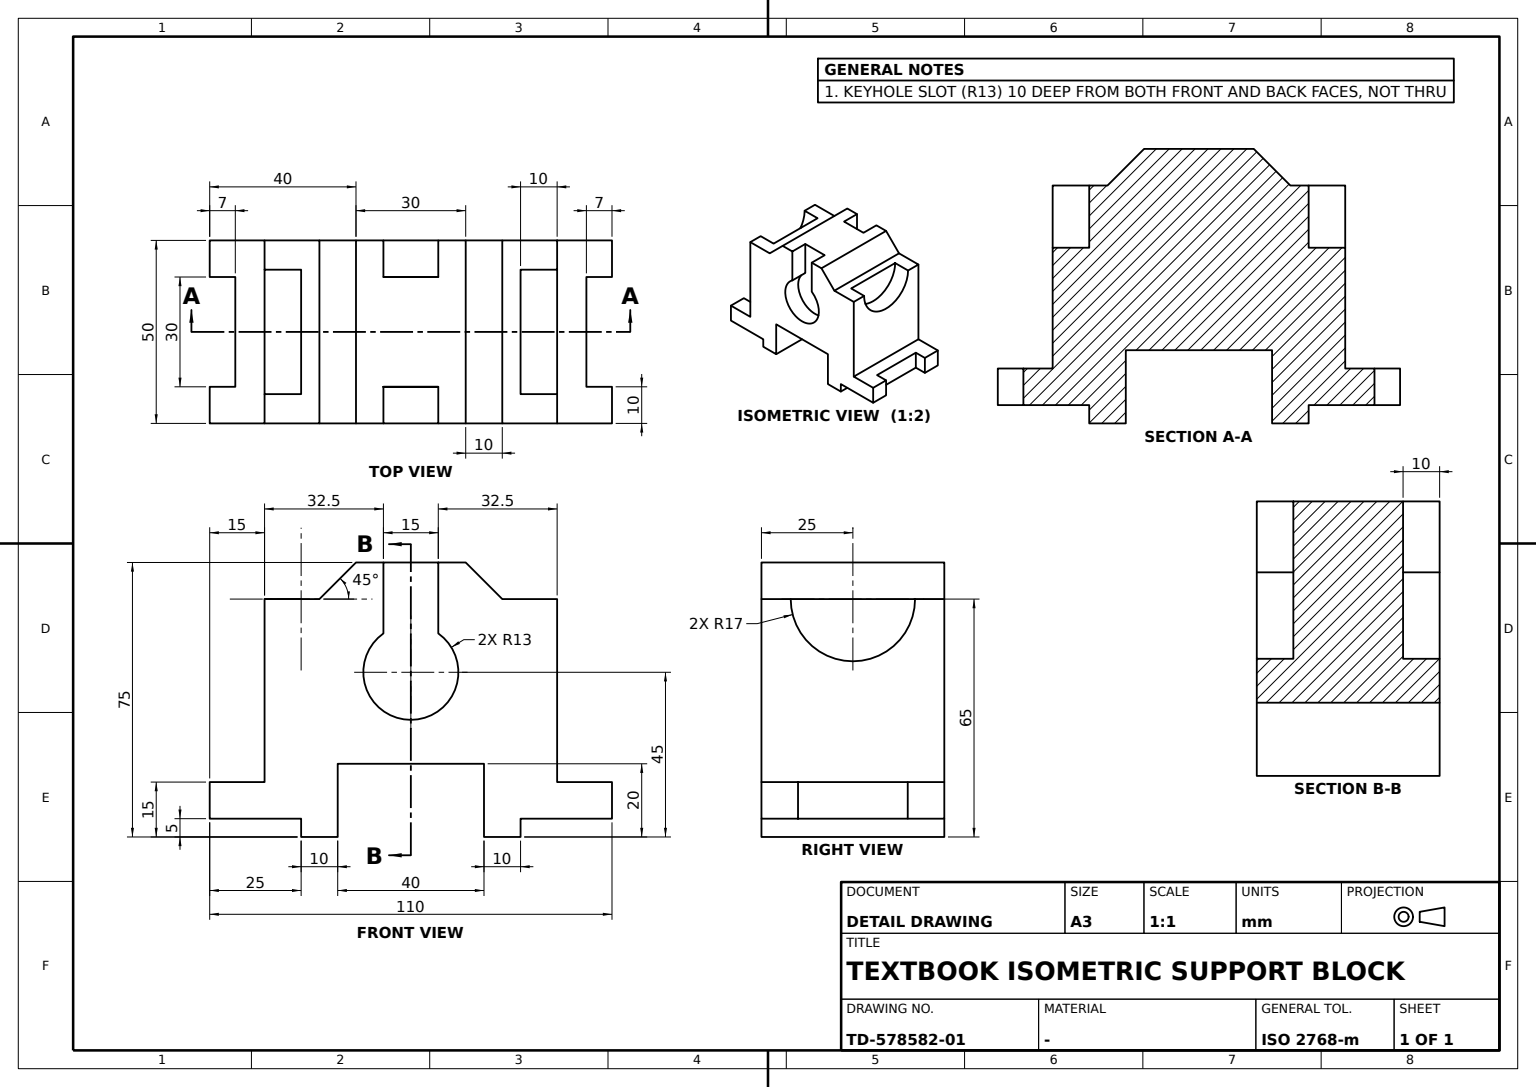
ISO-10303-21;
HEADER;
FILE_DESCRIPTION((''),'2;1');
FILE_NAME('','',(''),(''),'','','');
FILE_SCHEMA(('AUTOMOTIVE_DESIGN'));
ENDSEC;
DATA;
#1=APPLICATION_CONTEXT('');
#2=PRODUCT_CONTEXT('',#1,'mechanical');
#3=PRODUCT('','','',(#2));
#4=PRODUCT_DEFINITION_FORMATION('','',#3);
#5=PRODUCT_DEFINITION_CONTEXT('',#1,'design');
#6=PRODUCT_DEFINITION('','',#4,#5);
#7=PRODUCT_DEFINITION_SHAPE('','',#6);
#8=(LENGTH_UNIT()NAMED_UNIT(*)SI_UNIT(.MILLI.,.METRE.));
#9=(NAMED_UNIT(*)PLANE_ANGLE_UNIT()SI_UNIT($,.RADIAN.));
#10=(NAMED_UNIT(*)SI_UNIT($,.STERADIAN.)SOLID_ANGLE_UNIT());
#11=UNCERTAINTY_MEASURE_WITH_UNIT(LENGTH_MEASURE(0.005),#8,'distance_accuracy_value','');
#12=(GEOMETRIC_REPRESENTATION_CONTEXT(3)GLOBAL_UNCERTAINTY_ASSIGNED_CONTEXT((#11))GLOBAL_UNIT_ASSIGNED_CONTEXT((#8,#9,#10))REPRESENTATION_CONTEXT('',''));
#13=CARTESIAN_POINT('',(-78.,15.,5.));
#14=VERTEX_POINT('',#13);
#15=CARTESIAN_POINT('',(-78.,-15.,5.));
#16=VERTEX_POINT('',#15);
#17=CARTESIAN_POINT('',(-78.,0.,5.));
#18=DIRECTION('',(0.,-1.,0.));
#19=VECTOR('',#18,1000.);
#20=LINE('',#17,#19);
#21=EDGE_CURVE('',#14,#16,#20,.T.);
#22=ORIENTED_EDGE('',*,*,#21,.T.);
#23=CARTESIAN_POINT('',(-78.,-15.,15.));
#24=VERTEX_POINT('',#23);
#25=CARTESIAN_POINT('',(-78.,-15.,0.));
#26=DIRECTION('',(0.,0.,-1.));
#27=VECTOR('',#26,1000.);
#28=LINE('',#25,#27);
#29=EDGE_CURVE('',#24,#16,#28,.T.);
#30=ORIENTED_EDGE('',*,*,#29,.F.);
#31=CARTESIAN_POINT('',(-78.,15.,15.));
#32=VERTEX_POINT('',#31);
#33=LINE('',#31,#19);
#34=EDGE_CURVE('',#32,#24,#33,.T.);
#35=ORIENTED_EDGE('',*,*,#34,.F.);
#36=CARTESIAN_POINT('',(-78.,15.,0.));
#37=LINE('',#36,#27);
#38=EDGE_CURVE('',#32,#14,#37,.T.);
#39=ORIENTED_EDGE('',*,*,#38,.T.);
#40=EDGE_LOOP('',(#22,#30,#35,#39));
#41=FACE_BOUND('',#40,.T.);
#42=DIRECTION('',(1.,0.,0.));
#43=AXIS2_PLACEMENT_3D('',#31,#42,#18);
#44=PLANE('',#43);
#45=ADVANCED_FACE('',(#41),#44,.F.);
#46=ORIENTED_EDGE('',*,*,#21,.F.);
#47=CARTESIAN_POINT('',(-85.,15.,5.));
#48=VERTEX_POINT('',#47);
#49=CARTESIAN_POINT('',(0.,15.,5.));
#50=DIRECTION('',(-1.,0.,0.));
#51=VECTOR('',#50,1000.);
#52=LINE('',#49,#51);
#53=EDGE_CURVE('',#14,#48,#52,.T.);
#54=ORIENTED_EDGE('',*,*,#53,.T.);
#55=CARTESIAN_POINT('',(-85.,25.,5.));
#56=VERTEX_POINT('',#55);
#57=CARTESIAN_POINT('',(-85.,0.,5.));
#58=DIRECTION('',(0.,1.,0.));
#59=VECTOR('',#58,1000.);
#60=LINE('',#57,#59);
#61=EDGE_CURVE('',#48,#56,#60,.T.);
#62=ORIENTED_EDGE('',*,*,#61,.T.);
#63=CARTESIAN_POINT('',(-60.,25.,5.));
#64=VERTEX_POINT('',#63);
#65=CARTESIAN_POINT('',(0.,25.,5.));
#66=LINE('',#65,#51);
#67=EDGE_CURVE('',#64,#56,#66,.T.);
#68=ORIENTED_EDGE('',*,*,#67,.F.);
#69=CARTESIAN_POINT('',(-60.,-25.,5.));
#70=VERTEX_POINT('',#69);
#71=CARTESIAN_POINT('',(-60.,0.,5.));
#72=LINE('',#71,#59);
#73=EDGE_CURVE('',#70,#64,#72,.T.);
#74=ORIENTED_EDGE('',*,*,#73,.F.);
#75=CARTESIAN_POINT('',(-85.,-25.,5.));
#76=VERTEX_POINT('',#75);
#77=CARTESIAN_POINT('',(0.,-25.,5.));
#78=LINE('',#77,#51);
#79=EDGE_CURVE('',#70,#76,#78,.T.);
#80=ORIENTED_EDGE('',*,*,#79,.T.);
#81=CARTESIAN_POINT('',(-85.,-15.,5.));
#82=VERTEX_POINT('',#81);
#83=EDGE_CURVE('',#76,#82,#60,.T.);
#84=ORIENTED_EDGE('',*,*,#83,.T.);
#85=CARTESIAN_POINT('',(25.,-15.,5.));
#86=VECTOR('',#42,1000.);
#87=LINE('',#85,#86);
#88=EDGE_CURVE('',#82,#16,#87,.T.);
#89=ORIENTED_EDGE('',*,*,#88,.T.);
#90=EDGE_LOOP('',(#46,#54,#62,#68,#74,#80,#84,#89));
#91=FACE_BOUND('',#90,.T.);
#92=CARTESIAN_POINT('',(25.,0.,5.));
#93=AXIS2_PLACEMENT_3D('',#92,#26,#50);
#94=PLANE('',#93);
#95=ADVANCED_FACE('',(#91),#94,.T.);
#96=CARTESIAN_POINT('',(10.,-17.,65.));
#97=VERTEX_POINT('',#96);
#98=CARTESIAN_POINT('',(10.,17.,65.));
#99=VERTEX_POINT('',#98);
#100=CARTESIAN_POINT('',(10.,0.,65.));
#101=DIRECTION('',(0.,0.,1.));
#102=AXIS2_PLACEMENT_3D('',#100,#50,#101);
#103=CIRCLE('',#102,17.);
#104=EDGE_CURVE('',#97,#99,#103,.F.);
#105=ORIENTED_EDGE('',*,*,#104,.F.);
#106=CARTESIAN_POINT('',(10.,-25.,65.));
#107=VERTEX_POINT('',#106);
#108=LINE('',#100,#59);
#109=EDGE_CURVE('',#107,#97,#108,.T.);
#110=ORIENTED_EDGE('',*,*,#109,.F.);
#111=CARTESIAN_POINT('',(10.,-25.,15.));
#112=VERTEX_POINT('',#111);
#113=CARTESIAN_POINT('',(10.,-25.,0.));
#114=VECTOR('',#101,1000.);
#115=LINE('',#113,#114);
#116=EDGE_CURVE('',#112,#107,#115,.T.);
#117=ORIENTED_EDGE('',*,*,#116,.F.);
#118=CARTESIAN_POINT('',(10.,25.,15.));
#119=VERTEX_POINT('',#118);
#120=CARTESIAN_POINT('',(10.,0.,15.));
#121=LINE('',#120,#59);
#122=EDGE_CURVE('',#112,#119,#121,.T.);
#123=ORIENTED_EDGE('',*,*,#122,.T.);
#124=CARTESIAN_POINT('',(10.,25.,65.));
#125=VERTEX_POINT('',#124);
#126=CARTESIAN_POINT('',(10.,25.,0.));
#127=LINE('',#126,#114);
#128=EDGE_CURVE('',#119,#125,#127,.T.);
#129=ORIENTED_EDGE('',*,*,#128,.T.);
#130=EDGE_CURVE('',#99,#125,#108,.T.);
#131=ORIENTED_EDGE('',*,*,#130,.F.);
#132=EDGE_LOOP('',(#105,#110,#117,#123,#129,#131));
#133=FACE_BOUND('',#132,.T.);
#134=AXIS2_PLACEMENT_3D('',#120,#50,#101);
#135=PLANE('',#134);
#136=ADVANCED_FACE('',(#133),#135,.F.);
#137=CARTESIAN_POINT('',(-22.5,-15.,75.));
#138=VERTEX_POINT('',#137);
#139=CARTESIAN_POINT('',(-22.5,-15.,55.61838));
#140=VERTEX_POINT('',#139);
#141=LINE('',#137,#27);
#142=EDGE_CURVE('',#138,#140,#141,.T.);
#143=ORIENTED_EDGE('',*,*,#142,.T.);
#144=CARTESIAN_POINT('',(-22.5,-25.,55.61838));
#145=VERTEX_POINT('',#144);
#146=LINE('',#144,#59);
#147=EDGE_CURVE('',#145,#140,#146,.T.);
#148=ORIENTED_EDGE('',*,*,#147,.F.);
#149=CARTESIAN_POINT('',(-22.5,-25.,75.));
#150=VERTEX_POINT('',#149);
#151=LINE('',#149,#27);
#152=EDGE_CURVE('',#150,#145,#151,.T.);
#153=ORIENTED_EDGE('',*,*,#152,.F.);
#154=CARTESIAN_POINT('',(-22.5,0.,75.));
#155=LINE('',#154,#59);
#156=EDGE_CURVE('',#150,#138,#155,.T.);
#157=ORIENTED_EDGE('',*,*,#156,.T.);
#158=EDGE_LOOP('',(#143,#148,#153,#157));
#159=FACE_BOUND('',#158,.T.);
#160=CARTESIAN_POINT('',(-22.5,25.,75.));
#161=AXIS2_PLACEMENT_3D('',#160,#50,#26);
#162=PLANE('',#161);
#163=ADVANCED_FACE('',(#159),#162,.T.);
#164=CARTESIAN_POINT('',(-22.5,15.,55.61838));
#165=VERTEX_POINT('',#164);
#166=CARTESIAN_POINT('',(-37.5,15.,55.61838));
#167=VERTEX_POINT('',#166);
#168=CARTESIAN_POINT('',(-30.,15.,45.));
#169=AXIS2_PLACEMENT_3D('',#168,#58,#101);
#170=CIRCLE('',#169,13.);
#171=EDGE_CURVE('',#165,#167,#170,.T.);
#172=ORIENTED_EDGE('',*,*,#171,.F.);
#173=CARTESIAN_POINT('',(-22.5,25.,55.61838));
#174=VERTEX_POINT('',#173);
#175=LINE('',#173,#59);
#176=EDGE_CURVE('',#174,#165,#175,.F.);
#177=ORIENTED_EDGE('',*,*,#176,.F.);
#178=CARTESIAN_POINT('',(-37.5,25.,55.61838));
#179=VERTEX_POINT('',#178);
#180=CARTESIAN_POINT('',(-30.,25.,45.));
#181=AXIS2_PLACEMENT_3D('',#180,#58,#101);
#182=CIRCLE('',#181,13.);
#183=EDGE_CURVE('',#174,#179,#182,.T.);
#184=ORIENTED_EDGE('',*,*,#183,.T.);
#185=LINE('',#178,#59);
#186=EDGE_CURVE('',#179,#167,#185,.F.);
#187=ORIENTED_EDGE('',*,*,#186,.T.);
#188=EDGE_LOOP('',(#172,#177,#184,#187));
#189=FACE_BOUND('',#188,.T.);
#190=CARTESIAN_POINT('',(-30.,20.,45.));
#191=AXIS2_PLACEMENT_3D('',#190,#58,#50);
#192=CYLINDRICAL_SURFACE('',#191,13.);
#193=ADVANCED_FACE('',(#189),#192,.F.);
#194=CARTESIAN_POINT('',(-37.5,-15.,75.));
#195=VERTEX_POINT('',#194);
#196=CARTESIAN_POINT('',(0.,-15.,75.));
#197=LINE('',#196,#51);
#198=EDGE_CURVE('',#138,#195,#197,.T.);
#199=ORIENTED_EDGE('',*,*,#198,.T.);
#200=CARTESIAN_POINT('',(-37.5,-15.,55.61838));
#201=VERTEX_POINT('',#200);
#202=LINE('',#200,#114);
#203=EDGE_CURVE('',#201,#195,#202,.T.);
#204=ORIENTED_EDGE('',*,*,#203,.F.);
#205=CARTESIAN_POINT('',(-30.,-15.,45.));
#206=AXIS2_PLACEMENT_3D('',#205,#58,#101);
#207=CIRCLE('',#206,13.);
#208=EDGE_CURVE('',#140,#201,#207,.T.);
#209=ORIENTED_EDGE('',*,*,#208,.F.);
#210=ORIENTED_EDGE('',*,*,#142,.F.);
#211=EDGE_LOOP('',(#199,#204,#209,#210));
#212=FACE_BOUND('',#211,.T.);
#213=CARTESIAN_POINT('',(0.,-15.,0.));
#214=AXIS2_PLACEMENT_3D('',#213,#58,#50);
#215=PLANE('',#214);
#216=ADVANCED_FACE('',(#212),#215,.F.);
#217=CARTESIAN_POINT('',(25.,-25.,15.));
#218=VERTEX_POINT('',#217);
#219=CARTESIAN_POINT('',(25.,-15.,15.));
#220=VERTEX_POINT('',#219);
#221=CARTESIAN_POINT('',(25.,0.,15.));
#222=LINE('',#221,#59);
#223=EDGE_CURVE('',#218,#220,#222,.T.);
#224=ORIENTED_EDGE('',*,*,#223,.T.);
#225=CARTESIAN_POINT('',(18.,-15.,15.));
#226=VERTEX_POINT('',#225);
#227=CARTESIAN_POINT('',(-85.,-15.,15.));
#228=LINE('',#227,#51);
#229=EDGE_CURVE('',#220,#226,#228,.T.);
#230=ORIENTED_EDGE('',*,*,#229,.T.);
#231=CARTESIAN_POINT('',(18.,15.,15.));
#232=VERTEX_POINT('',#231);
#233=LINE('',#231,#19);
#234=EDGE_CURVE('',#232,#226,#233,.T.);
#235=ORIENTED_EDGE('',*,*,#234,.F.);
#236=CARTESIAN_POINT('',(25.,15.,15.));
#237=VERTEX_POINT('',#236);
#238=CARTESIAN_POINT('',(0.,15.,15.));
#239=LINE('',#238,#86);
#240=EDGE_CURVE('',#232,#237,#239,.T.);
#241=ORIENTED_EDGE('',*,*,#240,.T.);
#242=CARTESIAN_POINT('',(25.,25.,15.));
#243=VERTEX_POINT('',#242);
#244=EDGE_CURVE('',#237,#243,#222,.T.);
#245=ORIENTED_EDGE('',*,*,#244,.T.);
#246=CARTESIAN_POINT('',(-85.,25.,15.));
#247=LINE('',#246,#51);
#248=EDGE_CURVE('',#243,#119,#247,.T.);
#249=ORIENTED_EDGE('',*,*,#248,.T.);
#250=ORIENTED_EDGE('',*,*,#122,.F.);
#251=CARTESIAN_POINT('',(-85.,-25.,15.));
#252=LINE('',#251,#51);
#253=EDGE_CURVE('',#218,#112,#252,.T.);
#254=ORIENTED_EDGE('',*,*,#253,.F.);
#255=EDGE_LOOP('',(#224,#230,#235,#241,#245,#249,#250,#254));
#256=FACE_BOUND('',#255,.T.);
#257=CARTESIAN_POINT('',(-85.,0.,15.));
#258=AXIS2_PLACEMENT_3D('',#257,#101,#42);
#259=PLANE('',#258);
#260=ADVANCED_FACE('',(#256),#259,.T.);
#261=CARTESIAN_POINT('',(-60.,17.,65.));
#262=VERTEX_POINT('',#261);
#263=CARTESIAN_POINT('',(-60.,-17.,65.));
#264=VERTEX_POINT('',#263);
#265=CARTESIAN_POINT('',(-60.,0.,65.));
#266=AXIS2_PLACEMENT_3D('',#265,#50,#101);
#267=CIRCLE('',#266,17.);
#268=EDGE_CURVE('',#262,#264,#267,.T.);
#269=ORIENTED_EDGE('',*,*,#268,.T.);
#270=LINE('',#265,#19);
#271=EDGE_CURVE('',#262,#264,#270,.T.);
#272=ORIENTED_EDGE('',*,*,#271,.F.);
#273=EDGE_LOOP('',(#269,#272));
#274=FACE_BOUND('',#273,.T.);
#275=CARTESIAN_POINT('',(-60.,0.,0.));
#276=AXIS2_PLACEMENT_3D('',#275,#50,#101);
#277=PLANE('',#276);
#278=ADVANCED_FACE('',(#274),#277,.T.);
#279=CARTESIAN_POINT('',(-37.5,25.,75.));
#280=VERTEX_POINT('',#279);
#281=LINE('',#178,#114);
#282=EDGE_CURVE('',#179,#280,#281,.T.);
#283=ORIENTED_EDGE('',*,*,#282,.T.);
#284=CARTESIAN_POINT('',(-37.5,15.,75.));
#285=VERTEX_POINT('',#284);
#286=CARTESIAN_POINT('',(-37.5,0.,75.));
#287=LINE('',#286,#19);
#288=EDGE_CURVE('',#280,#285,#287,.T.);
#289=ORIENTED_EDGE('',*,*,#288,.T.);
#290=LINE('',#166,#114);
#291=EDGE_CURVE('',#167,#285,#290,.T.);
#292=ORIENTED_EDGE('',*,*,#291,.F.);
#293=ORIENTED_EDGE('',*,*,#186,.F.);
#294=EDGE_LOOP('',(#283,#289,#292,#293));
#295=FACE_BOUND('',#294,.T.);
#296=AXIS2_PLACEMENT_3D('',#178,#42,#101);
#297=PLANE('',#296);
#298=ADVANCED_FACE('',(#295),#297,.T.);
#299=CARTESIAN_POINT('',(18.,15.,5.));
#300=VERTEX_POINT('',#299);
#301=CARTESIAN_POINT('',(18.,-15.,5.));
#302=VERTEX_POINT('',#301);
#303=CARTESIAN_POINT('',(18.,0.,5.));
#304=LINE('',#303,#19);
#305=EDGE_CURVE('',#300,#302,#304,.T.);
#306=ORIENTED_EDGE('',*,*,#305,.F.);
#307=CARTESIAN_POINT('',(18.,15.,0.));
#308=LINE('',#307,#27);
#309=EDGE_CURVE('',#232,#300,#308,.T.);
#310=ORIENTED_EDGE('',*,*,#309,.F.);
#311=ORIENTED_EDGE('',*,*,#234,.T.);
#312=CARTESIAN_POINT('',(18.,-15.,0.));
#313=LINE('',#312,#27);
#314=EDGE_CURVE('',#226,#302,#313,.T.);
#315=ORIENTED_EDGE('',*,*,#314,.T.);
#316=EDGE_LOOP('',(#306,#310,#311,#315));
#317=FACE_BOUND('',#316,.T.);
#318=AXIS2_PLACEMENT_3D('',#231,#42,#18);
#319=PLANE('',#318);
#320=ADVANCED_FACE('',(#317),#319,.T.);
#321=VERTEX_POINT('',#160);
#322=LINE('',#160,#27);
#323=EDGE_CURVE('',#321,#174,#322,.T.);
#324=ORIENTED_EDGE('',*,*,#323,.T.);
#325=ORIENTED_EDGE('',*,*,#176,.T.);
#326=CARTESIAN_POINT('',(-22.5,15.,75.));
#327=VERTEX_POINT('',#326);
#328=LINE('',#326,#27);
#329=EDGE_CURVE('',#327,#165,#328,.T.);
#330=ORIENTED_EDGE('',*,*,#329,.F.);
#331=LINE('',#160,#19);
#332=EDGE_CURVE('',#321,#327,#331,.T.);
#333=ORIENTED_EDGE('',*,*,#332,.F.);
#334=EDGE_LOOP('',(#324,#325,#330,#333));
#335=FACE_BOUND('',#334,.T.);
#336=ADVANCED_FACE('',(#335),#162,.T.);
#337=CARTESIAN_POINT('',(25.,-25.,5.));
#338=VERTEX_POINT('',#337);
#339=VERTEX_POINT('',#77);
#340=EDGE_CURVE('',#338,#339,#78,.T.);
#341=ORIENTED_EDGE('',*,*,#340,.T.);
#342=VERTEX_POINT('',#65);
#343=CARTESIAN_POINT('',(0.,0.,5.));
#344=LINE('',#343,#59);
#345=EDGE_CURVE('',#339,#342,#344,.T.);
#346=ORIENTED_EDGE('',*,*,#345,.T.);
#347=CARTESIAN_POINT('',(25.,25.,5.));
#348=VERTEX_POINT('',#347);
#349=EDGE_CURVE('',#348,#342,#66,.T.);
#350=ORIENTED_EDGE('',*,*,#349,.F.);
#351=CARTESIAN_POINT('',(25.,15.,5.));
#352=VERTEX_POINT('',#351);
#353=LINE('',#92,#59);
#354=EDGE_CURVE('',#352,#348,#353,.T.);
#355=ORIENTED_EDGE('',*,*,#354,.F.);
#356=LINE('',#351,#86);
#357=EDGE_CURVE('',#300,#352,#356,.T.);
#358=ORIENTED_EDGE('',*,*,#357,.F.);
#359=ORIENTED_EDGE('',*,*,#305,.T.);
#360=VERTEX_POINT('',#85);
#361=CARTESIAN_POINT('',(0.,-15.,5.));
#362=LINE('',#361,#51);
#363=EDGE_CURVE('',#360,#302,#362,.T.);
#364=ORIENTED_EDGE('',*,*,#363,.F.);
#365=EDGE_CURVE('',#338,#360,#353,.T.);
#366=ORIENTED_EDGE('',*,*,#365,.F.);
#367=EDGE_LOOP('',(#341,#346,#350,#355,#358,#359,#364,#366));
#368=FACE_BOUND('',#367,.T.);
#369=ADVANCED_FACE('',(#368),#94,.T.);
#370=CARTESIAN_POINT('',(-70.,17.,65.));
#371=VERTEX_POINT('',#370);
#372=CARTESIAN_POINT('',(-70.,25.,65.));
#373=VERTEX_POINT('',#372);
#374=CARTESIAN_POINT('',(-70.,0.,65.));
#375=LINE('',#374,#59);
#376=EDGE_CURVE('',#371,#373,#375,.T.);
#377=ORIENTED_EDGE('',*,*,#376,.T.);
#378=CARTESIAN_POINT('',(-70.,25.,15.));
#379=VERTEX_POINT('',#378);
#380=CARTESIAN_POINT('',(-70.,25.,0.));
#381=LINE('',#380,#114);
#382=EDGE_CURVE('',#379,#373,#381,.T.);
#383=ORIENTED_EDGE('',*,*,#382,.F.);
#384=CARTESIAN_POINT('',(-70.,-25.,15.));
#385=VERTEX_POINT('',#384);
#386=CARTESIAN_POINT('',(-70.,0.,15.));
#387=LINE('',#386,#59);
#388=EDGE_CURVE('',#385,#379,#387,.T.);
#389=ORIENTED_EDGE('',*,*,#388,.F.);
#390=CARTESIAN_POINT('',(-70.,-25.,65.));
#391=VERTEX_POINT('',#390);
#392=CARTESIAN_POINT('',(-70.,-25.,0.));
#393=LINE('',#392,#114);
#394=EDGE_CURVE('',#385,#391,#393,.T.);
#395=ORIENTED_EDGE('',*,*,#394,.T.);
#396=CARTESIAN_POINT('',(-70.,-17.,65.));
#397=VERTEX_POINT('',#396);
#398=EDGE_CURVE('',#391,#397,#375,.T.);
#399=ORIENTED_EDGE('',*,*,#398,.T.);
#400=AXIS2_PLACEMENT_3D('',#374,#50,#101);
#401=CIRCLE('',#400,17.);
#402=EDGE_CURVE('',#371,#397,#401,.T.);
#403=ORIENTED_EDGE('',*,*,#402,.F.);
#404=EDGE_LOOP('',(#377,#383,#389,#395,#399,#403));
#405=FACE_BOUND('',#404,.T.);
#406=AXIS2_PLACEMENT_3D('',#386,#50,#101);
#407=PLANE('',#406);
#408=ADVANCED_FACE('',(#405),#407,.T.);
#409=ORIENTED_EDGE('',*,*,#329,.T.);
#410=ORIENTED_EDGE('',*,*,#171,.T.);
#411=ORIENTED_EDGE('',*,*,#291,.T.);
#412=CARTESIAN_POINT('',(0.,15.,75.));
#413=LINE('',#412,#51);
#414=EDGE_CURVE('',#327,#285,#413,.T.);
#415=ORIENTED_EDGE('',*,*,#414,.F.);
#416=EDGE_LOOP('',(#409,#410,#411,#415));
#417=FACE_BOUND('',#416,.T.);
#418=CARTESIAN_POINT('',(0.,15.,0.));
#419=AXIS2_PLACEMENT_3D('',#418,#58,#50);
#420=PLANE('',#419);
#421=ADVANCED_FACE('',(#417),#420,.T.);
#422=ORIENTED_EDGE('',*,*,#365,.T.);
#423=CARTESIAN_POINT('',(25.,-15.,0.));
#424=LINE('',#423,#27);
#425=EDGE_CURVE('',#220,#360,#424,.T.);
#426=ORIENTED_EDGE('',*,*,#425,.F.);
#427=ORIENTED_EDGE('',*,*,#223,.F.);
#428=CARTESIAN_POINT('',(25.,-25.,0.));
#429=LINE('',#428,#27);
#430=EDGE_CURVE('',#218,#338,#429,.T.);
#431=ORIENTED_EDGE('',*,*,#430,.T.);
#432=EDGE_LOOP('',(#422,#426,#427,#431));
#433=FACE_BOUND('',#432,.T.);
#434=AXIS2_PLACEMENT_3D('',#221,#42,#26);
#435=PLANE('',#434);
#436=ADVANCED_FACE('',(#433),#435,.T.);
#437=ORIENTED_EDGE('',*,*,#83,.F.);
#438=VERTEX_POINT('',#251);
#439=CARTESIAN_POINT('',(-85.,-25.,0.));
#440=LINE('',#439,#114);
#441=EDGE_CURVE('',#76,#438,#440,.T.);
#442=ORIENTED_EDGE('',*,*,#441,.T.);
#443=VERTEX_POINT('',#227);
#444=LINE('',#257,#59);
#445=EDGE_CURVE('',#438,#443,#444,.T.);
#446=ORIENTED_EDGE('',*,*,#445,.T.);
#447=LINE('',#81,#27);
#448=EDGE_CURVE('',#443,#82,#447,.T.);
#449=ORIENTED_EDGE('',*,*,#448,.T.);
#450=EDGE_LOOP('',(#437,#442,#446,#449));
#451=FACE_BOUND('',#450,.T.);
#452=AXIS2_PLACEMENT_3D('',#57,#50,#101);
#453=PLANE('',#452);
#454=ADVANCED_FACE('',(#451),#453,.T.);
#455=ORIENTED_EDGE('',*,*,#349,.T.);
#456=CARTESIAN_POINT('',(0.,25.,0.));
#457=VERTEX_POINT('',#456);
#458=LINE('',#456,#27);
#459=EDGE_CURVE('',#342,#457,#458,.T.);
#460=ORIENTED_EDGE('',*,*,#459,.T.);
#461=CARTESIAN_POINT('',(-10.,25.,0.));
#462=VERTEX_POINT('',#461);
#463=LINE('',#456,#51);
#464=EDGE_CURVE('',#457,#462,#463,.T.);
#465=ORIENTED_EDGE('',*,*,#464,.T.);
#466=CARTESIAN_POINT('',(-10.,25.,20.));
#467=VERTEX_POINT('',#466);
#468=LINE('',#461,#114);
#469=EDGE_CURVE('',#462,#467,#468,.T.);
#470=ORIENTED_EDGE('',*,*,#469,.T.);
#471=CARTESIAN_POINT('',(-50.,25.,20.));
#472=VERTEX_POINT('',#471);
#473=CARTESIAN_POINT('',(0.,25.,20.));
#474=LINE('',#473,#51);
#475=EDGE_CURVE('',#467,#472,#474,.T.);
#476=ORIENTED_EDGE('',*,*,#475,.T.);
#477=CARTESIAN_POINT('',(-50.,25.,0.));
#478=VERTEX_POINT('',#477);
#479=LINE('',#477,#27);
#480=EDGE_CURVE('',#472,#478,#479,.T.);
#481=ORIENTED_EDGE('',*,*,#480,.T.);
#482=CARTESIAN_POINT('',(-60.,25.,0.));
#483=VERTEX_POINT('',#482);
#484=EDGE_CURVE('',#478,#483,#463,.T.);
#485=ORIENTED_EDGE('',*,*,#484,.T.);
#486=LINE('',#482,#114);
#487=EDGE_CURVE('',#483,#64,#486,.T.);
#488=ORIENTED_EDGE('',*,*,#487,.T.);
#489=ORIENTED_EDGE('',*,*,#67,.T.);
#490=VERTEX_POINT('',#246);
#491=CARTESIAN_POINT('',(-85.,25.,0.));
#492=LINE('',#491,#114);
#493=EDGE_CURVE('',#56,#490,#492,.T.);
#494=ORIENTED_EDGE('',*,*,#493,.T.);
#495=CARTESIAN_POINT('',(0.,25.,15.));
#496=LINE('',#495,#86);
#497=EDGE_CURVE('',#490,#379,#496,.T.);
#498=ORIENTED_EDGE('',*,*,#497,.T.);
#499=ORIENTED_EDGE('',*,*,#382,.T.);
#500=CARTESIAN_POINT('',(-55.,25.,65.));
#501=VERTEX_POINT('',#500);
#502=CARTESIAN_POINT('',(0.,25.,65.));
#503=LINE('',#502,#86);
#504=EDGE_CURVE('',#373,#501,#503,.T.);
#505=ORIENTED_EDGE('',*,*,#504,.T.);
#506=CARTESIAN_POINT('',(-45.,25.,75.));
#507=VERTEX_POINT('',#506);
#508=CARTESIAN_POINT('',(-60.,25.,60.));
#509=DIRECTION('',(0.707106781,0.,0.707106781));
#510=VECTOR('',#509,1000.);
#511=LINE('',#508,#510);
#512=EDGE_CURVE('',#501,#507,#511,.T.);
#513=ORIENTED_EDGE('',*,*,#512,.T.);
#514=CARTESIAN_POINT('',(0.,25.,75.));
#515=LINE('',#514,#51);
#516=EDGE_CURVE('',#280,#507,#515,.T.);
#517=ORIENTED_EDGE('',*,*,#516,.F.);
#518=ORIENTED_EDGE('',*,*,#282,.F.);
#519=ORIENTED_EDGE('',*,*,#183,.F.);
#520=ORIENTED_EDGE('',*,*,#323,.F.);
#521=CARTESIAN_POINT('',(-15.,25.,75.));
#522=VERTEX_POINT('',#521);
#523=EDGE_CURVE('',#522,#321,#515,.T.);
#524=ORIENTED_EDGE('',*,*,#523,.F.);
#525=CARTESIAN_POINT('',(-5.,25.,65.));
#526=VERTEX_POINT('',#525);
#527=CARTESIAN_POINT('',(30.,25.,30.));
#528=DIRECTION('',(-0.707106781,0.,0.707106781));
#529=VECTOR('',#528,1000.);
#530=LINE('',#527,#529);
#531=EDGE_CURVE('',#526,#522,#530,.T.);
#532=ORIENTED_EDGE('',*,*,#531,.F.);
#533=LINE('',#372,#51);
#534=EDGE_CURVE('',#125,#526,#533,.T.);
#535=ORIENTED_EDGE('',*,*,#534,.F.);
#536=ORIENTED_EDGE('',*,*,#128,.F.);
#537=ORIENTED_EDGE('',*,*,#248,.F.);
#538=CARTESIAN_POINT('',(25.,25.,0.));
#539=LINE('',#538,#27);
#540=EDGE_CURVE('',#243,#348,#539,.T.);
#541=ORIENTED_EDGE('',*,*,#540,.T.);
#542=EDGE_LOOP('',(#455,#460,#465,#470,#476,#481,#485,#488,#489,#494,#498,#499,#505,#513,#517,#518,#519,#520,#524,#532,#535,#536,#537,#541));
#543=FACE_BOUND('',#542,.T.);
#544=AXIS2_PLACEMENT_3D('',#456,#58,#50);
#545=PLANE('',#544);
#546=ADVANCED_FACE('',(#543),#545,.T.);
#547=ORIENTED_EDGE('',*,*,#104,.T.);
#548=CARTESIAN_POINT('',(0.,17.,65.));
#549=VERTEX_POINT('',#548);
#550=LINE('',#548,#86);
#551=EDGE_CURVE('',#549,#99,#550,.T.);
#552=ORIENTED_EDGE('',*,*,#551,.F.);
#553=CARTESIAN_POINT('',(0.,-17.,65.));
#554=VERTEX_POINT('',#553);
#555=CARTESIAN_POINT('',(0.,0.,65.));
#556=AXIS2_PLACEMENT_3D('',#555,#42,#26);
#557=CIRCLE('',#556,17.);
#558=EDGE_CURVE('',#554,#549,#557,.T.);
#559=ORIENTED_EDGE('',*,*,#558,.F.);
#560=LINE('',#96,#86);
#561=EDGE_CURVE('',#97,#554,#560,.F.);
#562=ORIENTED_EDGE('',*,*,#561,.F.);
#563=EDGE_LOOP('',(#547,#552,#559,#562));
#564=FACE_BOUND('',#563,.T.);
#565=CARTESIAN_POINT('',(5.,0.,65.));
#566=AXIS2_PLACEMENT_3D('',#565,#42,#58);
#567=CYLINDRICAL_SURFACE('',#566,17.);
#568=ADVANCED_FACE('',(#564),#567,.F.);
#569=ORIENTED_EDGE('',*,*,#208,.T.);
#570=CARTESIAN_POINT('',(-37.5,-25.,55.61838));
#571=VERTEX_POINT('',#570);
#572=LINE('',#570,#59);
#573=EDGE_CURVE('',#571,#201,#572,.T.);
#574=ORIENTED_EDGE('',*,*,#573,.F.);
#575=CARTESIAN_POINT('',(-30.,-25.,45.));
#576=AXIS2_PLACEMENT_3D('',#575,#58,#101);
#577=CIRCLE('',#576,13.);
#578=EDGE_CURVE('',#145,#571,#577,.T.);
#579=ORIENTED_EDGE('',*,*,#578,.F.);
#580=ORIENTED_EDGE('',*,*,#147,.T.);
#581=EDGE_LOOP('',(#569,#574,#579,#580));
#582=FACE_BOUND('',#581,.T.);
#583=ADVANCED_FACE('',(#582),#192,.F.);
#584=ORIENTED_EDGE('',*,*,#29,.T.);
#585=ORIENTED_EDGE('',*,*,#88,.F.);
#586=ORIENTED_EDGE('',*,*,#448,.F.);
#587=CARTESIAN_POINT('',(0.,-15.,15.));
#588=LINE('',#587,#86);
#589=EDGE_CURVE('',#443,#24,#588,.T.);
#590=ORIENTED_EDGE('',*,*,#589,.T.);
#591=EDGE_LOOP('',(#584,#585,#586,#590));
#592=FACE_BOUND('',#591,.T.);
#593=ADVANCED_FACE('',(#592),#215,.T.);
#594=ORIENTED_EDGE('',*,*,#540,.F.);
#595=ORIENTED_EDGE('',*,*,#244,.F.);
#596=CARTESIAN_POINT('',(25.,15.,0.));
#597=LINE('',#596,#27);
#598=EDGE_CURVE('',#237,#352,#597,.T.);
#599=ORIENTED_EDGE('',*,*,#598,.T.);
#600=ORIENTED_EDGE('',*,*,#354,.T.);
#601=EDGE_LOOP('',(#594,#595,#599,#600));
#602=FACE_BOUND('',#601,.T.);
#603=ADVANCED_FACE('',(#602),#435,.T.);
#604=ORIENTED_EDGE('',*,*,#484,.F.);
#605=CARTESIAN_POINT('',(-50.,-25.,0.));
#606=VERTEX_POINT('',#605);
#607=CARTESIAN_POINT('',(-50.,0.,0.));
#608=LINE('',#607,#59);
#609=EDGE_CURVE('',#606,#478,#608,.T.);
#610=ORIENTED_EDGE('',*,*,#609,.F.);
#611=CARTESIAN_POINT('',(-60.,-25.,0.));
#612=VERTEX_POINT('',#611);
#613=CARTESIAN_POINT('',(0.,-25.,0.));
#614=LINE('',#613,#51);
#615=EDGE_CURVE('',#606,#612,#614,.T.);
#616=ORIENTED_EDGE('',*,*,#615,.T.);
#617=LINE('',#275,#59);
#618=EDGE_CURVE('',#612,#483,#617,.T.);
#619=ORIENTED_EDGE('',*,*,#618,.T.);
#620=EDGE_LOOP('',(#604,#610,#616,#619));
#621=FACE_BOUND('',#620,.T.);
#622=CARTESIAN_POINT('',(0.,0.,0.));
#623=AXIS2_PLACEMENT_3D('',#622,#26,#50);
#624=PLANE('',#623);
#625=ADVANCED_FACE('',(#621),#624,.T.);
#626=CARTESIAN_POINT('',(-10.,-25.,0.));
#627=VERTEX_POINT('',#626);
#628=CARTESIAN_POINT('',(-10.,0.,0.));
#629=LINE('',#628,#59);
#630=EDGE_CURVE('',#627,#462,#629,.T.);
#631=ORIENTED_EDGE('',*,*,#630,.T.);
#632=ORIENTED_EDGE('',*,*,#464,.F.);
#633=VERTEX_POINT('',#613);
#634=LINE('',#622,#59);
#635=EDGE_CURVE('',#633,#457,#634,.T.);
#636=ORIENTED_EDGE('',*,*,#635,.F.);
#637=EDGE_CURVE('',#633,#627,#614,.T.);
#638=ORIENTED_EDGE('',*,*,#637,.T.);
#639=EDGE_LOOP('',(#631,#632,#636,#638));
#640=FACE_BOUND('',#639,.T.);
#641=ADVANCED_FACE('',(#640),#624,.T.);
#642=CARTESIAN_POINT('',(-55.,-25.,65.));
#643=VERTEX_POINT('',#642);
#644=CARTESIAN_POINT('',(0.,-25.,65.));
#645=LINE('',#644,#86);
#646=EDGE_CURVE('',#391,#643,#645,.T.);
#647=ORIENTED_EDGE('',*,*,#646,.T.);
#648=CARTESIAN_POINT('',(-55.,0.,65.));
#649=LINE('',#648,#59);
#650=EDGE_CURVE('',#643,#501,#649,.T.);
#651=ORIENTED_EDGE('',*,*,#650,.T.);
#652=ORIENTED_EDGE('',*,*,#504,.F.);
#653=ORIENTED_EDGE('',*,*,#376,.F.);
#654=LINE('',#370,#86);
#655=EDGE_CURVE('',#371,#262,#654,.T.);
#656=ORIENTED_EDGE('',*,*,#655,.T.);
#657=ORIENTED_EDGE('',*,*,#271,.T.);
#658=LINE('',#263,#86);
#659=EDGE_CURVE('',#264,#397,#658,.F.);
#660=ORIENTED_EDGE('',*,*,#659,.T.);
#661=ORIENTED_EDGE('',*,*,#398,.F.);
#662=EDGE_LOOP('',(#647,#651,#652,#653,#656,#657,#660,#661));
#663=FACE_BOUND('',#662,.T.);
#664=AXIS2_PLACEMENT_3D('',#374,#101,#42);
#665=PLANE('',#664);
#666=ADVANCED_FACE('',(#663),#665,.T.);
#667=ORIENTED_EDGE('',*,*,#203,.T.);
#668=CARTESIAN_POINT('',(-37.5,-25.,75.));
#669=VERTEX_POINT('',#668);
#670=LINE('',#279,#59);
#671=EDGE_CURVE('',#669,#195,#670,.T.);
#672=ORIENTED_EDGE('',*,*,#671,.F.);
#673=LINE('',#570,#114);
#674=EDGE_CURVE('',#571,#669,#673,.T.);
#675=ORIENTED_EDGE('',*,*,#674,.F.);
#676=ORIENTED_EDGE('',*,*,#573,.T.);
#677=EDGE_LOOP('',(#667,#672,#675,#676));
#678=FACE_BOUND('',#677,.T.);
#679=ADVANCED_FACE('',(#678),#297,.T.);
#680=CARTESIAN_POINT('',(-5.,-25.,65.));
#681=VERTEX_POINT('',#680);
#682=CARTESIAN_POINT('',(-15.,-25.,75.));
#683=VERTEX_POINT('',#682);
#684=CARTESIAN_POINT('',(30.,-25.,30.));
#685=LINE('',#684,#529);
#686=EDGE_CURVE('',#681,#683,#685,.T.);
#687=ORIENTED_EDGE('',*,*,#686,.F.);
#688=CARTESIAN_POINT('',(-5.,0.,65.));
#689=LINE('',#688,#59);
#690=EDGE_CURVE('',#681,#526,#689,.T.);
#691=ORIENTED_EDGE('',*,*,#690,.T.);
#692=ORIENTED_EDGE('',*,*,#531,.T.);
#693=CARTESIAN_POINT('',(-15.,0.,75.));
#694=LINE('',#693,#59);
#695=EDGE_CURVE('',#683,#522,#694,.T.);
#696=ORIENTED_EDGE('',*,*,#695,.F.);
#697=EDGE_LOOP('',(#687,#691,#692,#696));
#698=FACE_BOUND('',#697,.T.);
#699=DIRECTION('',(-0.707106781,0.,-0.707106781));
#700=AXIS2_PLACEMENT_3D('',#688,#699,#528);
#701=PLANE('',#700);
#702=ADVANCED_FACE('',(#698),#701,.F.);
#703=CARTESIAN_POINT('',(-85.,15.,15.));
#704=VERTEX_POINT('',#703);
#705=LINE('',#703,#51);
#706=EDGE_CURVE('',#32,#704,#705,.T.);
#707=ORIENTED_EDGE('',*,*,#706,.F.);
#708=ORIENTED_EDGE('',*,*,#34,.T.);
#709=ORIENTED_EDGE('',*,*,#589,.F.);
#710=ORIENTED_EDGE('',*,*,#445,.F.);
#711=CARTESIAN_POINT('',(0.,-25.,15.));
#712=LINE('',#711,#86);
#713=EDGE_CURVE('',#438,#385,#712,.T.);
#714=ORIENTED_EDGE('',*,*,#713,.T.);
#715=ORIENTED_EDGE('',*,*,#388,.T.);
#716=ORIENTED_EDGE('',*,*,#497,.F.);
#717=EDGE_CURVE('',#704,#490,#444,.T.);
#718=ORIENTED_EDGE('',*,*,#717,.F.);
#719=EDGE_LOOP('',(#707,#708,#709,#710,#714,#715,#716,#718));
#720=FACE_BOUND('',#719,.T.);
#721=ADVANCED_FACE('',(#720),#259,.T.);
#722=CARTESIAN_POINT('',(-10.,-25.,20.));
#723=VERTEX_POINT('',#722);
#724=CARTESIAN_POINT('',(-10.,0.,20.));
#725=LINE('',#724,#59);
#726=EDGE_CURVE('',#723,#467,#725,.T.);
#727=ORIENTED_EDGE('',*,*,#726,.F.);
#728=CARTESIAN_POINT('',(-50.,-25.,20.));
#729=VERTEX_POINT('',#728);
#730=CARTESIAN_POINT('',(0.,-25.,20.));
#731=LINE('',#730,#51);
#732=EDGE_CURVE('',#723,#729,#731,.T.);
#733=ORIENTED_EDGE('',*,*,#732,.T.);
#734=CARTESIAN_POINT('',(-50.,0.,20.));
#735=LINE('',#734,#59);
#736=EDGE_CURVE('',#729,#472,#735,.T.);
#737=ORIENTED_EDGE('',*,*,#736,.T.);
#738=ORIENTED_EDGE('',*,*,#475,.F.);
#739=EDGE_LOOP('',(#727,#733,#737,#738));
#740=FACE_BOUND('',#739,.T.);
#741=AXIS2_PLACEMENT_3D('',#724,#26,#50);
#742=PLANE('',#741);
#743=ADVANCED_FACE('',(#740),#742,.T.);
#744=ORIENTED_EDGE('',*,*,#402,.T.);
#745=ORIENTED_EDGE('',*,*,#659,.F.);
#746=ORIENTED_EDGE('',*,*,#268,.F.);
#747=ORIENTED_EDGE('',*,*,#655,.F.);
#748=EDGE_LOOP('',(#744,#745,#746,#747));
#749=FACE_BOUND('',#748,.T.);
#750=ADVANCED_FACE('',(#749),#567,.F.);
#751=ORIENTED_EDGE('',*,*,#493,.F.);
#752=ORIENTED_EDGE('',*,*,#61,.F.);
#753=LINE('',#47,#27);
#754=EDGE_CURVE('',#704,#48,#753,.T.);
#755=ORIENTED_EDGE('',*,*,#754,.F.);
#756=ORIENTED_EDGE('',*,*,#717,.T.);
#757=EDGE_LOOP('',(#751,#752,#755,#756));
#758=FACE_BOUND('',#757,.T.);
#759=ADVANCED_FACE('',(#758),#453,.T.);
#760=ORIENTED_EDGE('',*,*,#551,.T.);
#761=ORIENTED_EDGE('',*,*,#130,.T.);
#762=ORIENTED_EDGE('',*,*,#534,.T.);
#763=ORIENTED_EDGE('',*,*,#690,.F.);
#764=LINE('',#390,#51);
#765=EDGE_CURVE('',#107,#681,#764,.T.);
#766=ORIENTED_EDGE('',*,*,#765,.F.);
#767=ORIENTED_EDGE('',*,*,#109,.T.);
#768=ORIENTED_EDGE('',*,*,#561,.T.);
#769=LINE('',#555,#19);
#770=EDGE_CURVE('',#549,#554,#769,.T.);
#771=ORIENTED_EDGE('',*,*,#770,.F.);
#772=EDGE_LOOP('',(#760,#761,#762,#763,#766,#767,#768,#771));
#773=FACE_BOUND('',#772,.T.);
#774=ADVANCED_FACE('',(#773),#665,.T.);
#775=ORIENTED_EDGE('',*,*,#736,.F.);
#776=LINE('',#605,#27);
#777=EDGE_CURVE('',#729,#606,#776,.T.);
#778=ORIENTED_EDGE('',*,*,#777,.T.);
#779=ORIENTED_EDGE('',*,*,#609,.T.);
#780=ORIENTED_EDGE('',*,*,#480,.F.);
#781=EDGE_LOOP('',(#775,#778,#779,#780));
#782=FACE_BOUND('',#781,.T.);
#783=AXIS2_PLACEMENT_3D('',#734,#42,#26);
#784=PLANE('',#783);
#785=ADVANCED_FACE('',(#782),#784,.T.);
#786=ORIENTED_EDGE('',*,*,#770,.T.);
#787=ORIENTED_EDGE('',*,*,#558,.T.);
#788=EDGE_LOOP('',(#786,#787));
#789=FACE_BOUND('',#788,.T.);
#790=AXIS2_PLACEMENT_3D('',#343,#42,#26);
#791=PLANE('',#790);
#792=ADVANCED_FACE('',(#789),#791,.T.);
#793=ORIENTED_EDGE('',*,*,#487,.F.);
#794=ORIENTED_EDGE('',*,*,#618,.F.);
#795=LINE('',#611,#114);
#796=EDGE_CURVE('',#612,#70,#795,.T.);
#797=ORIENTED_EDGE('',*,*,#796,.T.);
#798=ORIENTED_EDGE('',*,*,#73,.T.);
#799=EDGE_LOOP('',(#793,#794,#797,#798));
#800=FACE_BOUND('',#799,.T.);
#801=ADVANCED_FACE('',(#800),#277,.T.);
#802=ORIENTED_EDGE('',*,*,#357,.T.);
#803=ORIENTED_EDGE('',*,*,#598,.F.);
#804=ORIENTED_EDGE('',*,*,#240,.F.);
#805=ORIENTED_EDGE('',*,*,#309,.T.);
#806=EDGE_LOOP('',(#802,#803,#804,#805));
#807=FACE_BOUND('',#806,.T.);
#808=ADVANCED_FACE('',(#807),#420,.F.);
#809=ORIENTED_EDGE('',*,*,#345,.F.);
#810=LINE('',#613,#27);
#811=EDGE_CURVE('',#339,#633,#810,.T.);
#812=ORIENTED_EDGE('',*,*,#811,.T.);
#813=ORIENTED_EDGE('',*,*,#635,.T.);
#814=ORIENTED_EDGE('',*,*,#459,.F.);
#815=EDGE_LOOP('',(#809,#812,#813,#814));
#816=FACE_BOUND('',#815,.T.);
#817=ADVANCED_FACE('',(#816),#791,.T.);
#818=ORIENTED_EDGE('',*,*,#650,.F.);
#819=CARTESIAN_POINT('',(-45.,-25.,75.));
#820=VERTEX_POINT('',#819);
#821=CARTESIAN_POINT('',(-60.,-25.,60.));
#822=LINE('',#821,#510);
#823=EDGE_CURVE('',#643,#820,#822,.T.);
#824=ORIENTED_EDGE('',*,*,#823,.T.);
#825=CARTESIAN_POINT('',(-45.,0.,75.));
#826=LINE('',#825,#59);
#827=EDGE_CURVE('',#820,#507,#826,.T.);
#828=ORIENTED_EDGE('',*,*,#827,.T.);
#829=ORIENTED_EDGE('',*,*,#512,.F.);
#830=EDGE_LOOP('',(#818,#824,#828,#829));
#831=FACE_BOUND('',#830,.T.);
#832=AXIS2_PLACEMENT_3D('',#648,#528,#509);
#833=PLANE('',#832);
#834=ADVANCED_FACE('',(#831),#833,.T.);
#835=ORIENTED_EDGE('',*,*,#523,.T.);
#836=ORIENTED_EDGE('',*,*,#332,.T.);
#837=ORIENTED_EDGE('',*,*,#414,.T.);
#838=ORIENTED_EDGE('',*,*,#288,.F.);
#839=ORIENTED_EDGE('',*,*,#516,.T.);
#840=ORIENTED_EDGE('',*,*,#827,.F.);
#841=CARTESIAN_POINT('',(0.,-25.,75.));
#842=LINE('',#841,#51);
#843=EDGE_CURVE('',#669,#820,#842,.T.);
#844=ORIENTED_EDGE('',*,*,#843,.F.);
#845=ORIENTED_EDGE('',*,*,#671,.T.);
#846=ORIENTED_EDGE('',*,*,#198,.F.);
#847=ORIENTED_EDGE('',*,*,#156,.F.);
#848=EDGE_CURVE('',#683,#150,#842,.T.);
#849=ORIENTED_EDGE('',*,*,#848,.F.);
#850=ORIENTED_EDGE('',*,*,#695,.T.);
#851=EDGE_LOOP('',(#835,#836,#837,#838,#839,#840,#844,#845,#846,#847,#849,#850));
#852=FACE_BOUND('',#851,.T.);
#853=AXIS2_PLACEMENT_3D('',#693,#26,#50);
#854=PLANE('',#853);
#855=ADVANCED_FACE('',(#852),#854,.F.);
#856=ORIENTED_EDGE('',*,*,#79,.F.);
#857=ORIENTED_EDGE('',*,*,#796,.F.);
#858=ORIENTED_EDGE('',*,*,#615,.F.);
#859=ORIENTED_EDGE('',*,*,#777,.F.);
#860=ORIENTED_EDGE('',*,*,#732,.F.);
#861=LINE('',#626,#114);
#862=EDGE_CURVE('',#627,#723,#861,.T.);
#863=ORIENTED_EDGE('',*,*,#862,.F.);
#864=ORIENTED_EDGE('',*,*,#637,.F.);
#865=ORIENTED_EDGE('',*,*,#811,.F.);
#866=ORIENTED_EDGE('',*,*,#340,.F.);
#867=ORIENTED_EDGE('',*,*,#430,.F.);
#868=ORIENTED_EDGE('',*,*,#253,.T.);
#869=ORIENTED_EDGE('',*,*,#116,.T.);
#870=ORIENTED_EDGE('',*,*,#765,.T.);
#871=ORIENTED_EDGE('',*,*,#686,.T.);
#872=ORIENTED_EDGE('',*,*,#848,.T.);
#873=ORIENTED_EDGE('',*,*,#152,.T.);
#874=ORIENTED_EDGE('',*,*,#578,.T.);
#875=ORIENTED_EDGE('',*,*,#674,.T.);
#876=ORIENTED_EDGE('',*,*,#843,.T.);
#877=ORIENTED_EDGE('',*,*,#823,.F.);
#878=ORIENTED_EDGE('',*,*,#646,.F.);
#879=ORIENTED_EDGE('',*,*,#394,.F.);
#880=ORIENTED_EDGE('',*,*,#713,.F.);
#881=ORIENTED_EDGE('',*,*,#441,.F.);
#882=EDGE_LOOP('',(#856,#857,#858,#859,#860,#863,#864,#865,#866,#867,#868,#869,#870,#871,#872,#873,#874,#875,#876,#877,#878,#879,#880,#881));
#883=FACE_BOUND('',#882,.T.);
#884=AXIS2_PLACEMENT_3D('',#613,#58,#50);
#885=PLANE('',#884);
#886=ADVANCED_FACE('',(#883),#885,.F.);
#887=ORIENTED_EDGE('',*,*,#862,.T.);
#888=ORIENTED_EDGE('',*,*,#726,.T.);
#889=ORIENTED_EDGE('',*,*,#469,.F.);
#890=ORIENTED_EDGE('',*,*,#630,.F.);
#891=EDGE_LOOP('',(#887,#888,#889,#890));
#892=FACE_BOUND('',#891,.T.);
#893=AXIS2_PLACEMENT_3D('',#628,#50,#101);
#894=PLANE('',#893);
#895=ADVANCED_FACE('',(#892),#894,.T.);
#896=ORIENTED_EDGE('',*,*,#38,.F.);
#897=ORIENTED_EDGE('',*,*,#706,.T.);
#898=ORIENTED_EDGE('',*,*,#754,.T.);
#899=ORIENTED_EDGE('',*,*,#53,.F.);
#900=EDGE_LOOP('',(#896,#897,#898,#899));
#901=FACE_BOUND('',#900,.T.);
#902=ADVANCED_FACE('',(#901),#420,.F.);
#903=ORIENTED_EDGE('',*,*,#425,.T.);
#904=ORIENTED_EDGE('',*,*,#363,.T.);
#905=ORIENTED_EDGE('',*,*,#314,.F.);
#906=ORIENTED_EDGE('',*,*,#229,.F.);
#907=EDGE_LOOP('',(#903,#904,#905,#906));
#908=FACE_BOUND('',#907,.T.);
#909=ADVANCED_FACE('',(#908),#215,.T.);
#910=CLOSED_SHELL('',(#45,#95,#136,#163,#193,#216,#260,#278,#298,#320,#336,#369,#408,#421,#436,#454,#546,#568,#583,#593,#603,#625,#641,#666,#679,#702,#721,#743,#750,#759,#774,#785,#792,#801,#808,#817,#834,#855,#886,#895,#902,#909));
#911=MANIFOLD_SOLID_BREP('',#910);
#912=ADVANCED_BREP_SHAPE_REPRESENTATION('',(#911),#12);
#913=SHAPE_DEFINITION_REPRESENTATION(#7,#912);
ENDSEC;
END-ISO-10303-21;
